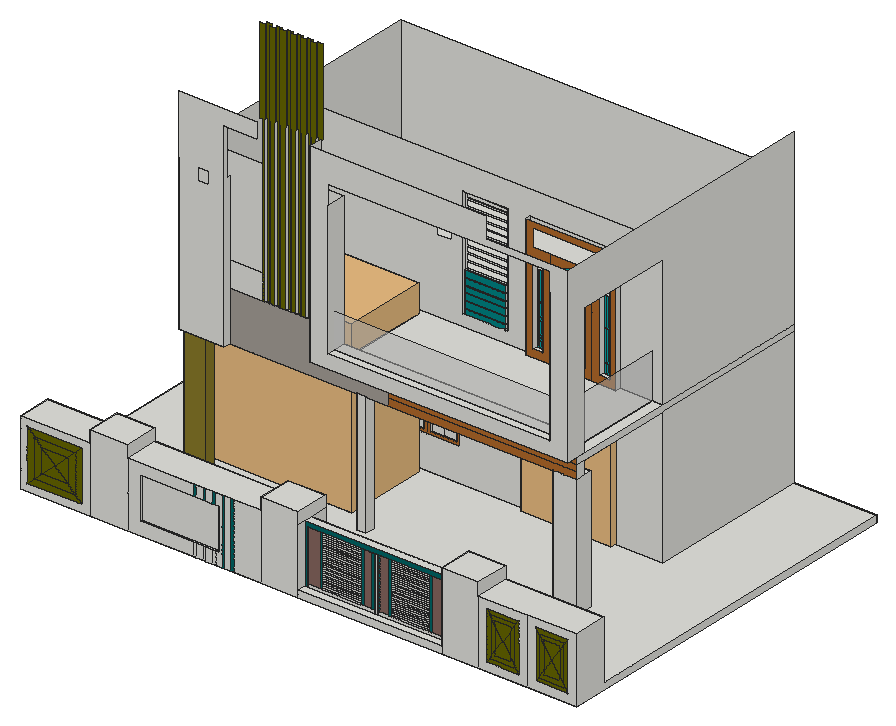
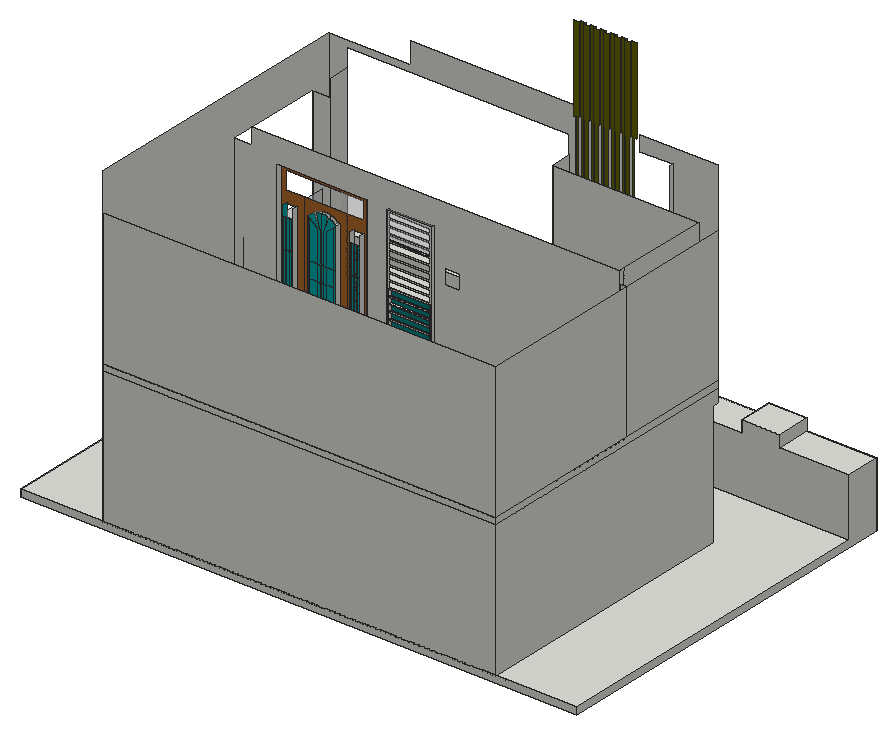
# SketchUp Ruby script. Lengths in inches.
U = 1.inch
M = Sketchup.active_model
def pt(a) = Geom::Point3d.new(a.map { |v| v * U })
def face(e, loops, mat)
  f = e.add_face(loops[0].map { |a| pt(a) })
  loops[1..].each { |l| e.add_face(l.map { |a| pt(a) }).erase! }
  f.material = f.back_material = mat if mat
  f
end
# faces: each face lists its corners as indices into pts; further lists are holes
def faces(e, pts, list, mat = nil) = list.each { |f| face(e, (f[0].is_a?(Array) ? f : [f]).map { |l| l.map { |i| pts[i] } }, mat) }
# xy, xz, yz: faces in a plane at the given z, y or x. An outline is a flat list of corners, or four numbers for a rectangle; further outlines are holes
def ring(l) = l.size == 4 ? [[l[0], l[1]], [l[2], l[1]], [l[2], l[3]], [l[0], l[3]]] : l.each_slice(2).to_a
def flat(e, list, mat, &to3) = list.each { |f| face(e, (f[0].is_a?(Array) ? f : [f]).map { |l| ring(l).map { |u, v| to3.(u, v) } }, mat) }
def xy(e, z, list, mat = nil) = flat(e, list, mat) { |x, y| [x, y, z] }
def xz(e, y, list, mat = nil) = flat(e, list, mat) { |x, z| [x, y, z] }
def yz(e, x, list, mat = nil) = flat(e, list, mat) { |y, z| [x, y, z] }
def lines(e, pts, list) = list.each { |a, b| e.add_line(pt(pts[a]), pt(pts[b])) }
# prism: a flat outline (further loops are holes) pulled along v
def prism(e, loops, v, mat = nil)
  f = face(e, loops, mat); d = Geom::Vector3d.new(v.map { |x| x * U })
  f.pushpull(f.normal.samedirection?(d) ? d.length : -d.length)
end
def box(e, o, s, mat = nil) = prism(e, [[o, [o[0] + s[0], o[1], o[2]], [o[0] + s[0], o[1] + s[1], o[2]], [o[0], o[1] + s[1], o[2]]]], [0, 0, s[2]], mat)
def at(x, y, z, deg = 0) = Geom::Transformation.translation(pt([x, y, z])) * Geom::Transformation.rotation(ORIGIN, Z_AXIS, deg.degrees)
def axes(o, x, y, z) = Geom::Transformation.new([*x, 0, *y, 0, *z, 0, *pt(o).to_a, 1])
def part(name) = M.definitions.add(name)
# library, detail: a bought-in or finely detailed component or shape, given as its bounding box
def library(name, o, s) = part(name).tap { |d| box(d.entities, o, s) }
def detail(e, o, s) = box(e.add_group.entities, o, s)
def put(e, d, t, mat = nil) = e.add_instance(d, t).tap { |i| i.material = mat if mat }
def group(e, t, mat = nil) = e.add_group.tap { |g| g.transformation = t; g.material = mat if mat }.entities
root = M.entities
M.materials.add("[Color E08]").color = [102, 102, 0]
M.materials.add("[Color H06]").color = [0, 170, 170]
M.materials.add("[Color H07]").color = [0, 132, 132]
M.materials.add("[Color H08]").color = [0, 102, 102]
M.materials.add("[Field Rectangle Tile]").color = [165, 159, 151]
M.materials.add("[Tile Mosaic Multi]").color = [135, 103, 96]
M.materials.add("[Translucent Glass Gray]").color = [209, 209, 209]
M.materials["[Translucent Glass Gray]"].alpha = 0.5
M.materials.add("[Wood Bamboo]").color = [177, 105, 43]
M.materials.add("[Wood Plywood Knots]").color = [137, 122, 41]
c1 = library("Group\#1",[0,0,0],[74.2,130.42,150.7])
c2 = library("Group\#2",[0,0,0],[80.4375,4.5,108.5625])
xy(root,-1.0625,[[0,0,494.5625,333.5625]])
xy(root,4.9375,[[247.28,0,374.58,7.27],[249.97,7.27,309.35,14.83],[309.35,7.27,311.98,14.83],[311.98,7.27,371.49,14.83],[[247.28,14.83,374.58,14.83,374.58,30.26,494.5625,30.26,494.5625,333.5625,421.0625,333.5625,421.0625,188.3125,77.78,188.3125,77.78,100.5,91.47,100.5,91.47,92.3125,71.6875,92.3125,71.6875,333.5625,0,333.5625,0,30.26,247.28,30.26],[399.51,92.3125,421.0625,108.18],[225.42,92.3125,233.79,100.5]],
  [71.6875,92.3125,91.47,92.3125,91.47,100.5,77.78,100.5,77.78,188.3125,421.0625,188.3125,421.0625,333.5625,71.6875,333.5625]])
xy(root,7.5,[[249.97,7.27,309.35,14.83],[311.98,7.27,371.49,14.83]])
xy(root,10.42,[[106.75,0,176.44,2]])
xy(root,37.14,[[185.11,188.3125,196.7,189.375],[196.7,188.3125,208.3,189.375],[214.36,188.3125,225.95,189.375],[225.95,188.3125,237.55,189.375]])
xy(root,47.04,[[106.75,0,176.44,2]])
xy(root,52.75,[[249.97,7.27,309.35,14.83],[309.35,7.27,311.98,14.83],[311.98,7.27,371.49,14.83]])
xy(root,56.875,[[0,0,61.54,30.26],[95.5625,0,214.14,30.26],[407.375,0,494.5625,30.26],[247.28,7.27,374.58,14.83]])
xy(root,67.375,[[61.54,0,95.5625,30.26],[214.14,0,247.28,30.26],[374.58,0,407.375,30.26]])
xy(root,83.87,[[185.11,188.3125,196.7,189.375],[196.7,188.3125,208.3,189.375],[214.36,188.3125,225.95,189.375],[225.95,188.3125,237.55,189.375]])
xy(root,88.73,[[183.91,188.3125,211.33,189.375],[211.33,188.3125,238.74,189.375]])
xy(root,98.22,[[183.91,188.3125,238.74,189.375]])
xy(root,113.5,[[71.6875,86.125,91.47,92.3125],[91.47,86.125,91.47,100.5,225.42,100.5,225.42,92.3125,112.4375,92.3125,112.4375,86.125],[225.42,92.3125,233.79,100.5],[233.79,92.3125,399.51,100.5],[399.51,92.3125,421.0625,100.5],
  [399.51,100.5,421.0625,108.18]])
xy(root,124.9375,[[207.78,100.5,207.78,183.18,77.78,183.18,77.78,188.3125,421.0625,188.3125,421.0625,100.5]])
xy(root,130.9375,[[191.8125,82.0625,421.0625,92.3125],[207.78,100.5,412.09,100.5,412.09,188.3125,382.89,188.3125,382.89,183.8125,302.45,183.8125,302.45,188.3125,77.78,188.3125,77.78,183.18,207.78,183.18],[412.09,100.5,421.0625,188.3125],[302.45,183.8125,302.45,188.3125,71.6875,188.3125,71.6875,333.5625,421.0625,333.5625,421.0625,188.3125,382.89,188.3125,382.89,183.8125]])
xy(root,137.87,[[308.71,183.8125,317.57,188.3125],[330.45,183.8125,354.72,188.3125],[368.2,183.8125,377.59,188.3125]])
xy(root,141.17,[[243.39,188.3125,244.9,190.25],[281.43,188.3125,282.95,190.25]])
xy(root,143.1875,[[207.78,82.0625,405.1875,89.12],[207.78,89.12,405.1875,100.5]])
xy(root,145.64,[[244.9,188.3125,281.43,190.25]])
xy(root,146.39,[[244.9,188.3125,281.43,190.25]])
xy(root,151.82,[[244.9,188.3125,281.43,190.25]])
xy(root,152.57,[[244.9,188.3125,281.43,190.25]])
xy(root,157.53,[[143.92,92.3125,148.41,94.5],[152.91,92.3125,157.41,94.5],[161.9,92.3125,166.4,94.5],[170.9,92.3125,175.4,94.5],[179.89,92.3125,184.39,94.5],
  [188.89,92.3125,191.8125,94.5]])
xy(root,158,[[244.9,188.3125,281.43,190.25]])
xy(root,158.75,[[244.9,188.3125,281.43,190.25]])
xy(root,164.19,[[244.9,188.3125,281.43,190.25]])
xy(root,164.94,[[244.9,188.3125,281.43,190.25]])
xy(root,170.37,[[244.9,188.3125,281.43,190.25]])
xy(root,171.12,[[244.9,188.3125,281.43,190.25]])
xz(root,0,[[[0,-1.0625,61.54,56.875],[6.11,5.05,55.42,50.76]],[61.54,-1.0625,95.5625,67.375],[95.5625,-1.0625,153.59,-1.0625,153.59,10.42,106.75,10.42,106.75,47.04,153.59,47.04,153.59,56.875,95.5625,56.875],[153.59,-1.0625,156.53,10.42],[156.53,-1.0625,162.21,10.42],
  [162.21,-1.0625,165.15,10.42],[165.15,-1.0625,170.65,10.42],[170.65,-1.0625,173.59,10.42],[173.59,-1.0625,178.9,-1.0625,178.9,56.875,173.59,56.875,173.59,47.04,176.44,47.04,176.44,10.42,173.59,10.42],[181.84,-1.0625,186.59,56.875],
  [189.53,-1.0625,214.14,56.875],[214.14,-1.0625,247.28,67.375],[247.28,-1.0625,374.58,4.9375],[374.58,-1.0625,407.375,67.375],[[407.375,-1.0625,450.97,56.875],[414.8,6.37,443.54,49.45]],
  [[450.97,-1.0625,494.5625,56.875],[458.4,6.37,487.13,49.45]],[156.53,47.04,162.21,56.875],[165.15,47.04,170.65,56.875]])
xz(root,0,[[6.11,5.05,12.71,11.17,12.23,11.17,12.23,44.65,12.71,44.65,6.11,50.76],[6.11,5.05,55.42,5.05,48.83,11.17,12.71,11.17],[55.42,5.05,55.42,50.76,48.83,44.65,49.31,44.65,49.31,11.17,48.83,11.17],[414.8,6.37,418.55,11.99,418.55,43.82,414.8,49.45],[414.8,6.37,443.54,6.37,439.79,11.99,439.79,10.12,418.55,10.12,418.55,11.99],
  [443.54,6.37,443.54,49.45,439.79,43.82,439.79,11.99],[458.4,6.37,462.15,11.99,462.15,43.82,458.4,49.45],[458.4,6.37,487.13,6.37,483.38,11.99,483.38,10.12,462.15,10.12,462.15,11.99],[487.13,6.37,487.13,49.45,483.38,43.82,483.38,11.99],[418.55,10.12,439.79,10.12,439.79,11.99,436.04,17.61,436.04,13.87,422.31,13.87,422.31,17.61,418.55,11.99],
  [462.15,10.12,483.38,10.12,483.38,11.99,479.63,17.61,479.63,13.87,465.9,13.87,465.9,17.61,462.15,11.99],[12.23,11.17,12.71,11.17,19.3,17.28,18.34,17.28,18.34,38.53,19.3,38.53,12.71,44.65,12.23,44.65],[12.71,11.17,48.83,11.17,42.23,17.28,19.3,17.28],[48.83,11.17,49.31,11.17,49.31,44.65,48.83,44.65,42.23,38.53,43.2,38.53,43.2,17.28,42.23,17.28],[418.55,11.99,422.31,17.61,422.31,38.2,418.55,43.82],
  [439.79,11.99,439.79,43.82,436.04,38.2,436.04,17.61],[462.15,11.99,465.9,17.61,465.9,38.2,462.15,43.82],[483.38,11.99,483.38,43.82,479.63,38.2,479.63,17.61],[422.31,13.87,436.04,13.87,436.04,17.61,429.17,27.91,422.31,17.61],[465.9,13.87,479.63,13.87,479.63,17.61,472.77,27.91,465.9,17.61],
  [18.34,17.28,19.3,17.28,30.77,27.91,19.3,38.53,18.34,38.53],[19.3,17.28,42.23,17.28,30.77,27.91],[42.23,17.28,43.2,17.28,43.2,38.53,42.23,38.53,30.77,27.91],[422.31,17.61,429.17,27.91,422.31,38.2],[436.04,17.61,436.04,38.2,429.17,27.91],
  [465.9,17.61,472.77,27.91,465.9,38.2],[479.63,17.61,479.63,38.2,472.77,27.91],[30.77,27.91,42.23,38.53,19.3,38.53],[429.17,27.91,436.04,38.2,436.04,41.94,422.31,41.94,422.31,38.2],[472.77,27.91,479.63,38.2,479.63,41.94,465.9,41.94,465.9,38.2],
  [422.31,38.2,422.31,41.94,436.04,41.94,436.04,38.2,439.79,43.82,439.79,45.7,418.55,45.7,418.55,43.82],[465.9,38.2,465.9,41.94,479.63,41.94,479.63,38.2,483.38,43.82,483.38,45.7,462.15,45.7,462.15,43.82],[19.3,38.53,42.23,38.53,48.83,44.65,12.71,44.65],[418.55,43.82,418.55,45.7,439.79,45.7,439.79,43.82,443.54,49.45,414.8,49.45],[462.15,43.82,462.15,45.7,483.38,45.7,483.38,43.82,487.13,49.45,458.4,49.45],
  [12.71,44.65,48.83,44.65,55.42,50.76,6.11,50.76]],"[Color E08]")
xz(root,0,[[178.9,-1.0625,181.84,56.875],[186.59,-1.0625,189.53,56.875],[153.59,47.04,156.53,56.875],[162.21,47.04,165.15,56.875],[170.65,47.04,173.59,56.875]],"[Color H08]")
xz(root,2,[[106.75,10.42,176.44,47.04]])
xz(root,7.27,[[249.97,4.9375,309.35,7.5],[309.35,4.9375,311.98,52.75],[311.98,4.9375,371.49,7.5],[263.22,7.5,297.35,9.01],[324.53,7.5,357.62,9.01],
  [263.22,9.01,297.35,10.52],[324.53,9.01,357.62,10.52],[263.22,10.52,297.35,12.03],[324.53,10.52,357.62,12.03],[263.22,12.03,297.35,13.54],
  [324.53,12.03,357.62,13.54],[263.22,13.54,297.35,15.04],[324.53,13.54,357.62,15.04],[263.22,15.04,297.35,16.55],[324.53,15.04,357.62,16.55],
  [263.22,16.55,297.35,18.06],[324.53,16.55,357.62,18.06],[263.22,18.06,297.35,19.57],[324.53,18.06,357.62,19.57],[263.22,19.57,297.35,21.08],
  [324.53,19.57,357.62,21.08],[263.22,21.08,297.35,22.58],[324.53,21.08,357.62,22.58],[263.22,22.58,297.35,24.09],[324.53,22.58,357.62,24.09],
  [263.22,24.09,297.35,25.6],[324.53,24.09,357.62,25.6],[263.22,25.6,297.35,27.11],[324.53,25.6,357.62,27.11],[263.22,27.11,297.35,28.62],
  [324.53,27.11,357.62,28.62],[263.22,28.62,297.35,30.125],[324.53,28.62,357.62,30.125],[263.22,30.125,297.35,31.63],[324.53,30.125,357.62,31.63],
  [263.22,31.63,297.35,33.14],[324.53,31.63,357.62,33.14],[263.22,33.14,297.35,34.65],[324.53,33.14,357.62,34.65],[263.22,34.65,297.35,36.16],
  [324.53,34.65,357.62,36.16],[263.22,36.16,297.35,37.67],[324.53,36.16,357.62,37.67],[263.22,37.67,297.35,39.18],[324.53,37.67,357.62,39.18],
  [263.22,39.18,297.35,40.68],[324.53,39.18,357.62,40.68],[263.22,40.68,297.35,42.19],[324.53,40.68,357.62,42.19],[263.22,42.19,297.35,43.7],
  [324.53,42.19,357.62,43.7],[263.22,43.7,297.35,45.21],[324.53,43.7,357.62,45.21],[263.22,45.21,297.35,46.72],[324.53,45.21,357.62,46.72],
  [263.22,46.72,297.35,48.23],[324.53,46.72,357.62,48.23],[263.22,48.23,297.35,49.73],[324.53,48.23,357.62,49.73],[263.22,49.73,297.35,51.24],
  [324.53,49.73,357.62,51.24],[263.22,51.24,297.35,52.75],[324.53,51.24,357.62,52.75]])
xz(root,7.27,[[247.28,4.9375,249.97,4.9375,249.97,52.75,371.49,52.75,371.49,4.9375,374.58,4.9375,374.58,56.875,247.28,56.875],[261.04,7.5,263.22,52.75],[297.35,7.5,299.53,52.75],[307.17,7.5,309.35,52.75],[311.98,7.5,314.15,52.75],
  [322.35,7.5,324.53,52.75],[357.62,7.5,359.98,52.75]],"[Color H08]")
xz(root,7.27,[[249.97,7.5,261.04,52.75],[299.53,7.5,307.17,52.75],[314.15,7.5,322.35,52.75],[359.98,7.5,371.49,52.75]],"[Tile Mosaic Multi]")
xz(root,14.83,[[247.28,4.9375,249.97,56.875],[249.97,4.9375,309.35,7.5],[371.49,4.9375,371.49,52.75,249.97,52.75,249.97,56.875,373.59,56.875,373.59,4.9375],[309.35,4.9375,311.98,52.75],[311.98,4.9375,371.49,7.5],
  [373.59,4.9375,374.58,56.875]])
xz(root,30.26,[[0,4.9375,0,56.875,61.54,56.875,61.54,67.375,95.5625,67.375,95.5625,56.875,214.14,56.875,214.14,67.375,247.28,67.375,247.28,4.9375],[374.58,4.9375,374.58,67.375,407.375,67.375,407.375,56.875,494.5625,56.875,494.5625,4.9375]])
xz(root,82.0625,[[[191.8125,130.9375,421.0625,130.9375,421.0625,284.3125,348.59,284.3125,348.59,303,191.8125,303],[207.78,143.1875,405.1875,278.6875]]])
xz(root,86.125,[[[71.6875,113.5,112.4375,113.5,112.4375,289.375,141.5625,289.375,141.5625,303,71.6875,303],[89.43,237.5,98.55,249]]])
xz(root,89.12,[[207.78,143.1875,405.1875,174.49]],"[Translucent Glass Gray]")
xz(root,92.3125,[[225.42,4.9375,233.79,113.5],[399.51,4.9375,421.0625,113.5],[112.4375,157.53,141.5625,179.96]])
xz(root,92.3125,[[141.5625,157.53,143.92,157.53,143.92,379.625,139.42,379.625,139.42,303,141.5625,303],[148.41,157.53,152.91,379.625],[157.41,157.53,161.9,379.625],[166.4,157.53,170.9,379.625],[175.4,157.53,179.89,379.625],
  [184.39,157.53,188.89,379.625]],"[Color E08]")
xz(root,92.3125,[[112.4375,113.5,252.91,113.5,252.91,130.9375,191.8125,130.9375,191.8125,157.53,112.4375,157.53]],"[Field Rectangle Tile]")
xz(root,92.3125,[[252.91,113.5,421.0625,119.3125],[252.91,119.3125,421.0625,125.125],[252.91,125.125,421.0625,130.9375]],"[Wood Bamboo]")
xz(root,92.3125,[[71.6875,4.9375,91.47,113.5]],"[Wood Plywood Knots]")
xz(root,94.5,[[143.92,157.53,148.41,379.625],[152.91,157.53,157.41,379.625],[161.9,157.53,166.4,379.625],[170.9,157.53,175.4,379.625],[179.89,157.53,184.39,379.625],
  [188.89,157.53,191.8125,157.53,191.8125,303,193.38,303,193.38,379.625,188.89,379.625]],"[Color E08]")
xz(root,100.5,[[77.78,4.9375,91.47,113.5],[225.42,4.9375,233.79,113.5],[77.78,113.5,207.78,130.9375],[207.78,113.5,421.0625,124.9375],[77.78,130.9375,207.78,261.3125],
  [207.78,130.9375,405.1875,143.1875],[405.1875,130.9375,421.0625,245.8125]])
xz(root,108.18,[[399.51,4.9375,421.0625,113.5]])
xz(root,183.18,[[77.78,124.9375,207.78,130.9375]])
xz(root,183.8125,[[[302.45,130.9375,323.52,130.9375,323.52,218.86,308.45,218.86,308.45,234.3,378.32,234.3,378.32,218.86,361.65,218.86,361.65,130.9375,382.89,130.9375,382.89,239.5,302.45,239.5],[368.2,137.87,377.59,208.65],[308.71,137.87,317.57,207.99]],[[323.52,130.9375,361.65,218.86],[330.45,137.87,330.45,207.99,332.04,209.68,333.85,211.12,335.26,211.93,335.86,212.27,338.02,213.12,340.28,213.63,342.59,213.8,344.9,213.63,347.16,213.12,349.32,212.27,349.92,211.93,351.33,211.12,353.14,209.68,354.72,207.99,354.72,137.87]]],"[Wood Bamboo]")
xz(root,188.3125,[[[77.78,4.9375,421.0625,124.9375],[182.08,34.12,240.58,100.05]],[71.6875,130.9375,77.78,250.9375],[[77.78,130.9375,302.45,130.9375,302.45,239.5,382.89,239.5,382.89,130.9375,421.0625,130.9375,421.0625,246.5625,405.1875,246.5625,405.1875,261.3125,77.78,261.3125],[243.39,141.17,282.95,238.98],[219.45,195.85,232.76,209.16]]])
xz(root,188.3125,[[308.71,137.87,309.6,146.35],[309.6,137.87,310.48,146.35],[310.48,137.87,311.37,146.35],[311.37,137.87,312.26,146.35],[312.26,137.87,313.14,146.35],
  [313.14,137.87,314.03,146.35],[314.03,137.87,314.91,146.35],[314.91,137.87,315.8,146.35],[315.8,137.87,316.6875,146.35],[316.6875,137.87,317.57,146.35],
  [330.45,137.87,332.06,172.93],[332.06,137.87,339.16,145.17],[339.16,137.87,340.84,145.17],[340.84,137.87,342.59,145.17],[342.59,137.87,344.28,145.17],
  [344.28,137.87,346.22,145.17],[346.22,137.87,353.11,145.17],[353.11,137.87,354.72,172.93],[368.2,137.87,369.24,146.35],[369.24,137.87,370.28,146.35],
  [370.28,137.87,371.33,146.35],[371.33,137.87,372.37,146.35],[372.37,137.87,373.41,146.35],[373.41,137.87,374.46,146.35],[374.46,137.87,375.5,146.35],
  [375.5,137.87,376.54,146.35],[376.54,137.87,377.59,146.35],[332.06,145.17,339.16,158.66],[339.16,145.17,340.84,158.66],[340.84,145.17,342.59,158.66],
  [342.59,145.17,344.28,158.66],[344.28,145.17,346.22,158.66],[346.22,145.17,353.11,158.66],[308.71,146.35,309.6,174.22],[309.6,146.35,310.48,174.22],
  [310.48,146.35,311.37,174.22],[311.37,146.35,312.26,174.22],[312.26,146.35,313.14,174.22],[313.14,146.35,314.03,174.22],[314.03,146.35,314.91,174.22],
  [314.91,146.35,315.8,174.22],[315.8,146.35,316.6875,174.22],[316.6875,146.35,317.57,174.22],[368.2,146.35,369.24,174.22],[369.24,146.35,370.28,174.22],
  [370.28,146.35,371.33,174.22],[371.33,146.35,372.37,174.22],[372.37,146.35,373.41,174.22],[373.41,146.35,374.46,174.22],[374.46,146.35,375.5,174.22],
  [375.5,146.35,376.54,174.22],[376.54,146.35,377.59,174.22],[332.06,158.66,339.16,172.93],[339.16,158.66,340.84,172.93],[340.84,158.66,342.59,172.93],
  [342.59,158.66,344.28,172.93],[344.28,158.66,346.22,172.93],[346.22,158.66,353.11,172.93],[330.45,172.93,332.06,172.93,332.06,206.7,330.45,207.99],[339.16,172.93,340.84,172.93,340.84,199.63,336.4,212.48,335.86,212.27,335.26,211.93,333.85,211.12,332.04,209.68,330.45,207.99,332.06,206.7,339.16,200.99],
  [332.06,172.93,339.16,172.93,339.16,200.99,332.06,206.7],[340.84,172.93,342.59,172.93,342.59,213.8,340.28,213.63,338.02,213.12,340.84,199.63],[342.59,172.93,344.28,172.93,344.28,199.63,347.16,213.12,344.9,213.63,342.59,213.8],[344.28,172.93,346.22,172.93,346.22,201.18,353.11,206.7,354.72,207.99,353.14,209.68,351.33,211.12,349.92,211.93,349.32,212.27,344.28,199.63],[346.22,172.93,353.11,172.93,353.11,206.7,346.22,201.18],
  [353.11,172.93,354.72,172.93,354.72,207.99,353.11,206.7],[308.71,174.22,309.6,199.67],[309.6,174.22,310.48,199.67],[310.48,174.22,311.37,199.67],[311.37,174.22,312.26,199.67],
  [312.26,174.22,313.14,199.67],[313.14,174.22,314.03,199.67],[314.03,174.22,314.91,199.67],[314.91,174.22,315.8,199.67],[315.8,174.22,316.6875,199.67],
  [316.6875,174.22,317.57,199.67],[368.2,174.22,369.24,199.91],[369.24,174.22,370.28,199.91],[370.28,174.22,371.33,199.91],[371.33,174.22,372.37,199.91],
  [372.37,174.22,373.41,199.91],[373.41,174.22,374.46,199.91],[374.46,174.22,375.5,199.91],[375.5,174.22,376.54,199.91],[376.54,174.22,377.59,199.91]],"[Color H06]")
xz(root,188.3125,[[244.9,141.17,281.43,145.64],[244.9,146.39,281.43,151.82],[244.9,152.57,281.43,158],[244.9,158.75,281.43,164.19],[244.9,164.94,281.43,170.37],
  [244.9,171.12,281.43,176.55]],"[Color H07]")
xz(root,188.3125,[[[182.08,34.12,211.33,86.9],[185.11,37.14,208.3,83.87]],[[211.33,34.12,240.58,86.9],[214.36,37.14,237.55,83.87]],[[182.08,86.9,240.58,100.05],[183.91,88.73,238.74,98.22]]],"[Wood Bamboo]")
xz(root,189.375,[[185.11,37.14,196.7,60.51],[196.7,37.14,208.3,60.51],[214.36,37.14,225.95,60.51],[225.95,37.14,237.55,60.51],[185.11,60.51,196.7,83.87],
  [196.7,60.51,208.3,83.87],[214.36,60.51,225.95,83.87],[225.95,60.51,237.55,83.87],[183.91,88.73,238.74,98.22]])
xz(root,190.25,[[[243.39,141.17,244.9,141.17,244.9,145.64,281.43,145.64,281.43,141.17,282.95,141.17,282.95,238.98,243.39,238.98],[244.9,164.94,281.43,170.37],[244.9,208.22,281.43,213.65],[244.9,146.39,281.43,151.82],[244.9,152.57,281.43,158],[244.9,177.3,281.43,182.73],[244.9,183.48,281.43,188.92],[244.9,189.67,281.43,195.1],[244.9,195.85,281.43,201.28],[244.9,220.58,281.43,226.02],[244.9,226.77,281.43,232.2],[244.9,158.75,281.43,164.19],[244.9,171.12,281.43,176.55],[244.9,202.03,281.43,207.47],[244.9,214.4,281.43,219.83],[244.9,232.95,281.43,237.47]]])
xz(root,333.5625,[[0,-1.0625,494.5625,4.9375],[71.6875,4.9375,421.0625,124.9375],[71.6875,124.9375,421.0625,130.9375],[71.6875,130.9375,421.0625,250.9375]])
yz(root,0,[[0,-1.0625,0,56.875,30.26,56.875,30.26,4.9375,333.5625,4.9375,333.5625,-1.0625]])
yz(root,61.54,[[0,56.875,30.26,67.375]])
yz(root,71.6875,[[92.3125,4.9375,92.3125,113.5,86.125,113.5,86.125,124.9375,333.5625,124.9375,333.5625,4.9375],[86.125,124.9375,333.5625,130.9375],[86.125,130.9375,188.3125,250.9375],[188.3125,130.9375,333.5625,250.9375]])
yz(root,77.78,[[100.5,4.9375,188.3125,124.9375],[100.5,124.9375,183.18,130.9375],[100.5,130.9375,183.18,261.3125],[183.18,130.9375,188.3125,261.3125]])
yz(root,91.47,[[92.3125,4.9375,100.5,113.5]],"[Wood Plywood Knots]")
yz(root,95.5625,[[0,56.875,30.26,67.375]])
yz(root,106.75,[[0,10.42,2,47.04]])
yz(root,112.4375,[[86.125,113.5,92.3125,113.5,92.3125,247.25,89,247.25,89,289.375,86.125,289.375]])
yz(root,143.92,[[92.3125,157.53,94.5,303]])
yz(root,148.41,[[92.3125,157.53,94.5,303]])
yz(root,152.91,[[92.3125,157.53,94.5,303]])
yz(root,157.41,[[92.3125,157.53,94.5,303]])
yz(root,161.9,[[92.3125,157.53,94.5,303]])
yz(root,166.4,[[92.3125,157.53,94.5,303]])
yz(root,170.9,[[92.3125,157.53,94.5,303]])
yz(root,175.4,[[92.3125,157.53,94.5,303]])
yz(root,176.44,[[0,10.42,2,47.04]])
yz(root,179.89,[[92.3125,157.53,94.5,303]])
yz(root,183.91,[[188.3125,88.73,189.375,98.22]])
yz(root,184.39,[[92.3125,157.53,94.5,303]])
yz(root,185.11,[[188.3125,37.14,189.375,83.87]])
yz(root,188.89,[[92.3125,157.53,94.5,303]])
yz(root,191.8125,[[82.0625,130.9375,82.0625,303,94.5,303,94.5,157.53,92.3125,157.53,92.3125,130.9375]])
yz(root,207.78,[[100.5,124.9375,183.18,130.9375],[82.0625,143.1875,100.5,261.3125]])
yz(root,208.3,[[188.3125,37.14,189.375,83.87]])
yz(root,214.14,[[0,56.875,30.26,67.375]])
yz(root,214.36,[[188.3125,37.14,189.375,83.87]])
yz(root,225.42,[[92.3125,4.9375,100.5,113.5]])
yz(root,233.79,[[92.3125,4.9375,100.5,113.5]])
yz(root,237.55,[[188.3125,37.14,189.375,83.87]])
yz(root,238.74,[[188.3125,88.73,189.375,98.22]])
yz(root,243.39,[[188.3125,141.17,190.25,238.98]])
yz(root,244.9,[[188.3125,141.17,190.25,142.69],[188.3125,142.69,190.25,145.64],[188.3125,146.39,190.25,151.82],[188.3125,152.57,190.25,158],[188.3125,158.75,190.25,164.19],
  [188.3125,164.94,190.25,170.37],[188.3125,171.12,190.25,176.55]])
yz(root,247.28,[[0,4.9375,7.27,56.875],[14.83,4.9375,30.26,56.875],[0,56.875,30.26,67.375]])
yz(root,249.97,[[7.27,4.9375,14.83,7.5],[7.27,7.5,14.83,52.75]])
yz(root,281.43,[[188.3125,141.17,190.25,142.69],[188.3125,142.69,190.25,145.64],[188.3125,146.39,190.25,151.82],[188.3125,152.57,190.25,158],[188.3125,158.75,190.25,164.19],
  [188.3125,164.94,190.25,170.37],[188.3125,171.12,190.25,176.55]])
yz(root,282.95,[[188.3125,141.17,190.25,238.98]])
yz(root,302.45,[[183.8125,130.9375,188.3125,239.5]])
yz(root,308.71,[[183.8125,137.87,188.3125,207.99]])
yz(root,309.35,[[7.27,4.9375,14.83,7.5],[7.27,7.5,14.83,52.75]])
yz(root,311.98,[[7.27,4.9375,14.83,7.5],[7.27,7.5,14.83,52.75]])
yz(root,317.57,[[183.8125,137.87,188.3125,207.99]])
yz(root,330.45,[[183.8125,137.87,188.3125,207.99]])
yz(root,354.72,[[183.8125,137.87,188.3125,207.99]])
yz(root,368.2,[[183.8125,137.87,188.3125,208.65]])
yz(root,371.49,[[7.27,4.9375,14.83,7.5],[7.27,7.5,14.83,52.75]])
yz(root,374.58,[[0,4.9375,0,67.375,30.26,67.375,30.26,4.9375,14.83,4.9375,14.83,56.875,7.27,56.875,7.27,4.9375]])
yz(root,377.59,[[183.8125,137.87,188.3125,208.65]],"[Color H06]")
yz(root,382.89,[[183.8125,130.9375,188.3125,239.5]])
yz(root,399.51,[[92.3125,4.9375,108.18,113.5]])
yz(root,405.1875,[[82.0625,143.1875,100.5,261.3125]])
yz(root,407.375,[[0,56.875,30.26,67.375]])
yz(root,412.09,[[100.5,130.9375,188.3125,170.96]],"[Translucent Glass Gray]")
yz(root,421.0625,[[92.3125,4.9375,108.18,113.5],[188.3125,4.9375,333.5625,124.9375],[92.3125,113.5,100.5,124.9375],[92.3125,124.9375,333.5625,130.9375],[82.0625,130.9375,100.5,130.9375,100.5,246.5625,188.3125,246.5625,188.3125,130.9375,333.5625,130.9375,333.5625,284.3125,82.0625,284.3125]])
yz(root,494.5625,[[0,-1.0625,333.5625,-1.0625,333.5625,4.9375,30.26,4.9375,30.26,56.875,0,56.875]])
p = [[77.78,100.5,124.9375],[77.78,92.3125,124.9375],[206.77,144.18,34.9375],[206.77,144.18,40.9375]]
lines(root,p,[[0,1],[2,3]])
put(root,c1,at(207.78,109.03,4.9375,90))
put(root,c2,at(298.18,183.8125,4.9375))
